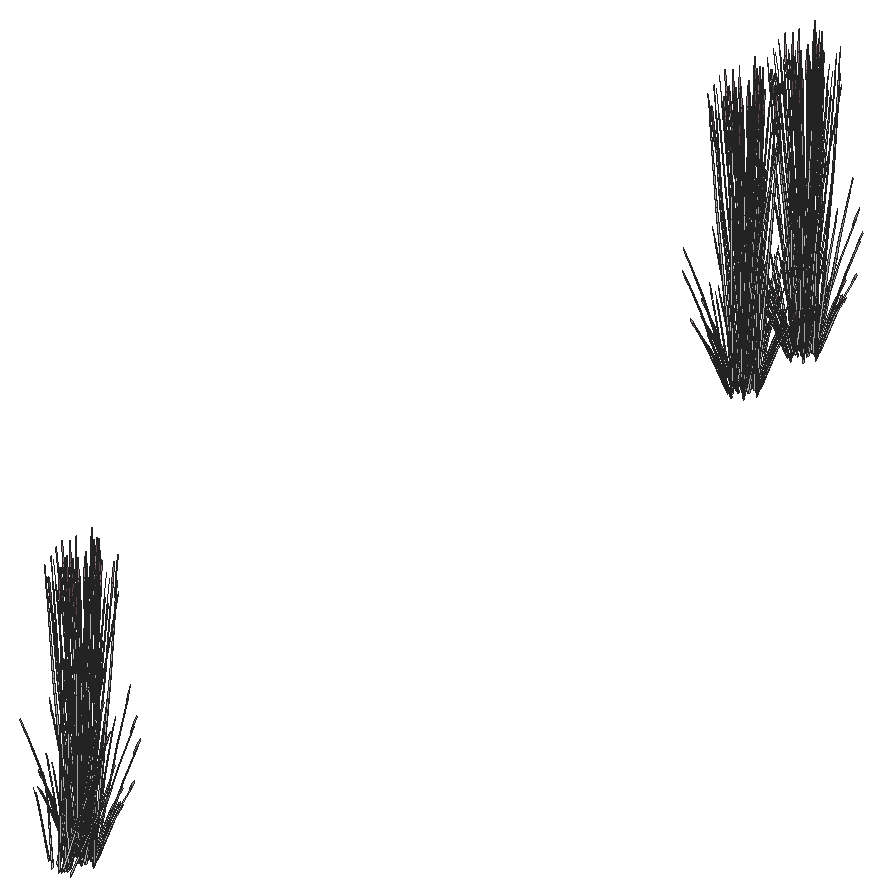
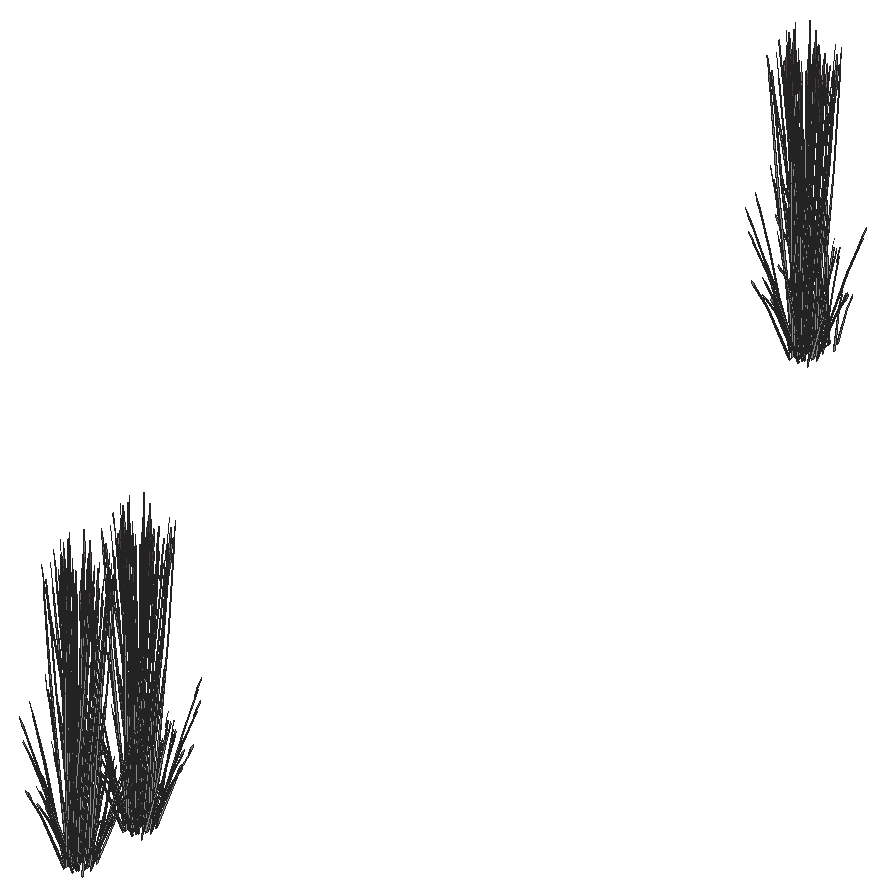
# SketchUp Ruby script. Lengths in inches.
U = 1.inch
M = Sketchup.active_model
def pt(a) = Geom::Point3d.new(a.map { |v| v * U })
def face(e, loops, mat)
  f = e.add_face(loops[0].map { |a| pt(a) })
  loops[1..].each { |l| e.add_face(l.map { |a| pt(a) }).erase! }
  f.material = f.back_material = mat if mat
  f
end
# faces: each face lists its corners as indices into pts; further lists are holes
def faces(e, pts, list, mat = nil) = list.each { |f| face(e, (f[0].is_a?(Array) ? f : [f]).map { |l| l.map { |i| pts[i] } }, mat) }
# xy, xz, yz: faces in a plane at the given z, y or x. An outline is a flat list of corners, or four numbers for a rectangle; further outlines are holes
def ring(l) = l.size == 4 ? [[l[0], l[1]], [l[2], l[1]], [l[2], l[3]], [l[0], l[3]]] : l.each_slice(2).to_a
def flat(e, list, mat, &to3) = list.each { |f| face(e, (f[0].is_a?(Array) ? f : [f]).map { |l| ring(l).map { |u, v| to3.(u, v) } }, mat) }
def xy(e, z, list, mat = nil) = flat(e, list, mat) { |x, y| [x, y, z] }
def xz(e, y, list, mat = nil) = flat(e, list, mat) { |x, z| [x, y, z] }
def yz(e, x, list, mat = nil) = flat(e, list, mat) { |y, z| [x, y, z] }
def lines(e, pts, list) = list.each { |a, b| e.add_line(pt(pts[a]), pt(pts[b])) }
# prism: a flat outline (further loops are holes) pulled along v
def prism(e, loops, v, mat = nil)
  f = face(e, loops, mat); d = Geom::Vector3d.new(v.map { |x| x * U })
  f.pushpull(f.normal.samedirection?(d) ? d.length : -d.length)
end
def box(e, o, s, mat = nil) = prism(e, [[o, [o[0] + s[0], o[1], o[2]], [o[0] + s[0], o[1] + s[1], o[2]], [o[0], o[1] + s[1], o[2]]]], [0, 0, s[2]], mat)
def at(x, y, z, deg = 0) = Geom::Transformation.translation(pt([x, y, z])) * Geom::Transformation.rotation(ORIGIN, Z_AXIS, deg.degrees)
def axes(o, x, y, z) = Geom::Transformation.new([*x, 0, *y, 0, *z, 0, *pt(o).to_a, 1])
def part(name) = M.definitions.add(name)
# library, detail: a bought-in or finely detailed component or shape, given as its bounding box
def library(name, o, s) = part(name).tap { |d| box(d.entities, o, s) }
def detail(e, o, s) = box(e.add_group.entities, o, s)
def put(e, d, t, mat = nil) = e.add_instance(d, t).tap { |i| i.material = mat if mat }
def group(e, t, mat = nil) = e.add_group.tap { |g| g.transformation = t; g.material = mat if mat }.entities
root = M.entities
M.materials.add("LightPink_Translucent").color = [144, 107, 117]
M.materials["LightPink_Translucent"].alpha = 0.75
c1 = part("blade")
p = [[2.15,0.21,22],[0,0.17,0],[0.09,0.45,0],[2.18,0.31,22],[2.29,0.31,22],[0.38,0.45,0],
  [2.48,0.24,33],[2.49,0.24,33],[2.48,0.22,33]]
faces(c1.entities,p,[[0,1,2,3],[4,5,2,3],[6,3,4,7],[8,0,3,6]])
c2 = part("seeds")
p = [[0.3,-0.1,1.38],[-0.01,-0.03,1.59],[-0.01,-0.03,0.03],[0.14,-0.07,-0.07],[0.29,-0.03,3],[0.15,0.01,3.11]]
faces(c2.entities,p,[[0,1,2,3],[1,0,4,5]],"LightPink_Translucent")
c3 = part("blade with seeds")
put(c3.entities,c1,at(0,0,0))
put(c3.entities,c2,axes([2.4,0.25,30.99],[1.5799,-0.05474,1.17369],[-0.12525,1.92788,0.29478],[-0.07173,-0.02425,1.56792]))
put(root,c3,axes([426.58,488.27,152.34],[0.17079,-0.21377,0.97034],[0.06739,0.33841,0.71294],[-0.12342,0.0606,0.21373]))
put(root,c3,axes([428.38,490.95,152],[-0.25622,-0.47263,0],[0.42866,-0.26357,-0.43598],[0.09763,-0.06003,1.38303]))
put(root,c3,axes([429.57,487.08,152.25],[0.04775,0.53819,-0.2458],[-0.49736,0.03254,-0.42242],[-0.08758,0.07169,1.34921]))
put(root,c3,axes([428.95,490.38,151.8],[-0.28319,0.27058,-0.03288],[-0.25948,-0.29635,-0.1491],[-0.01827,-0.08397,0.4918]))
put(root,c3,axes([429.76,488.09,151.97],[0.51304,0.1533,0.25983],[-0.12835,0.54797,-0.30828],[-0.08491,0.06858,1.39295]))
put(root,c3,axes([431.01,491.7,152.1875],[-0.1464,-0.01397,1.20808],[-0.14998,-0.37477,-0.25981],[0.17985,-0.10602,0.51652]))
put(root,c3,axes([431.18,491.01,152.34],[-0.1365,0.2401,0.97034],[-0.11733,-0.32258,0.71294],[0.11274,-0.08083,0.21373]))
put(root,c3,axes([430.42,488.04,152.34],[-0.23074,-0.13562,0.97034],[0.29794,-0.1378,0.71294],[0.08036,0.11673,0.21373]))
put(root,c3,axes([428.89,492.26,152.25],[-0.04775,-0.53819,-0.2458],[0.49736,-0.03254,-0.42242],[0.08758,-0.07169,1.34921]))
put(root,c3,axes([430.08,488.39,152],[0.25622,0.47263,0],[-0.42866,0.26357,-0.43598],[-0.09763,0.06003,1.38303]))
put(root,c3,axes([427.54,490.875,151.8],[-0.11822,0.38513,-0.03288],[-0.36385,-0.11847,-0.1491],[-0.05524,-0.06299,0.4918]))
put(root,c3,axes([430.48,488.55,151.26],[0.02986,-0.06809,1.48974],[0.37589,-0.20055,-0.22758],[0.11396,0.1038,0.25375]))
put(root,c3,axes([428.66,492.82,152.25],[-0.46151,-0.22505,-0.2458],[0.22222,-0.475,-0.42242],[-0.0145,-0.11662,1.34921]))
put(root,c3,axes([429.86,486.52,152.4],[-0.01119,-0.44408,1.19347],[0.50665,0.11511,0.50532],[-0.11983,0.243,1.12654]))
put(root,c3,axes([427.03,488.49,151.26],[0.05497,0.04712,1.48974],[0.09321,0.43661,-0.22758],[-0.12183,0.0931,0.25375]))
put(root,c3,axes([427.34,492.63,152],[-0.51243,0,0],[0,-0.52715,-0.43598],[0,-0.12006,1.38303]))
put(root,c3,axes([427.43,491.69,152.1875],[0.08001,0.13132,1.20808],[-0.18437,0.35694,-0.25981],[-0.18931,-0.08532,0.51652]))
put(root,c3,axes([430.46,488.66,152.25],[-0.26279,-0.01479,0.88755],[0.17355,-0.31417,0.49003],[0.10382,0.11162,0.6962]))
put(root,c3,axes([427.74,492.5,151.97],[-0.38118,0.39654,0.25983],[-0.38142,-0.39237,-0.30828],[-0.01331,-0.11261,1.39295]))
put(root,c3,axes([429.6,487.9,152.1875],[0.00723,-0.15635,1.20808],[0.34559,-0.17464,-0.25981],[0.10668,0.18713,0.51652]))
put(root,c3,axes([428.95,492.68,152.06],[0.46174,0.2286,0.2033],[-0.22222,0.475,0.42242],[0,-0.1095,1.35626]))
put(root,c3,axes([428.77,493.32,152.06],[0.10862,-0.55889,-0.19793],[0.515,0.09742,0.43313],[-0.08999,-0.07718,1.32161]))
put(root,c3,axes([428.03,489.2,152.34],[-0.01061,-0.28045,0.97034],[0.26501,0.20003,0.71294],[-0.05212,0.13367,0.21373]))
put(root,c3,axes([426.95,492.09,152.34],[0.26163,-0.03375,0.97034],[-0.16596,0.29737,0.71294],[-0.12929,-0.04461,0.21373]))
put(root,c3,axes([428.73,488.53,151.26],[0.06632,-0.02567,1.48974],[0.39894,0.14126,-0.22758],[0.01167,0.15921,0.25375]))
put(root,c3,axes([428.8,492.36,152.3],[-0.44501,0.02912,0.37796],[-0.04024,-0.48332,-0.1819],[0.07967,-0.04899,1.2135]))
put(root,c3,axes([427.65,492.71,152.09],[0,0.47166,0.41945],[-0.45849,0,0],[0,-0.10742,1.33059]))
put(root,c3,axes([430.27,491.07,152.01],[0.25622,-0.47263,0],[0.42866,0.26357,-0.43598],[0.09763,0.06003,1.38303]))
put(root,c3,axes([428.79,492.54,151.99],[0.17817,0.52741,0.38653],[-0.50909,0.1834,0.15168],[0.00622,-0.09691,1.34202]))
put(root,c3,axes([427.8125,488.6,152.38],[0.37228,-0.08352,0.05498],[0.08559,0.3365,-0.7291],[-0.0236,0.17034,0.65354]))
put(root,c3,axes([431.28,492.94,151.67],[-0.26394,0.0566,1.1961],[-0.04201,-0.45055,0.06846],[0.18486,-0.06819,0.68062]))
put(root,c3,axes([431.76,492.54,151.91],[-0.25407,-0.3016,-0.05481],[0.27826,-0.27635,-0.2485],[0.07884,-0.01946,0.81966]))
put(root,c3,axes([428.7,492.95,152.3],[-0.19883,0.425,0.37796],[-0.41314,-0.20454,-0.1819],[0,-0.09797,1.2135]))
put(root,c3,axes([429.43,492.58,151.86],[0,-0.54574,0],[0.51243,0,0],[0,0,1.51605]))
put(root,c3,axes([430.05,491.32,152.09],[-0.38354,-0.23583,0.41945],[0.22925,-0.42288,0],[0.08735,0.05371,1.33059]))
put(root,c3,axes([429.18,492.24,151.99],[-0.33979,0.42804,0.38653],[-0.40368,-0.37784,0.15168],[0.08192,-0.04272,1.34202]))
put(root,c3,axes([429.56,493,151.94],[-0.38118,-0.40596,-0.0518],[0.38142,-0.40621,0],[-0.01331,-0.01418,1.48322]))
put(root,c3,axes([428.59,491.53,152.09],[-0.11838,0.46875,0.14904],[-0.43321,-0.13265,0.29641],[0.07483,-0.00228,1.35512]))
put(root,c3,axes([428.42,491.91,151.35],[-0.40337,0.18883,1.08919],[-0.12839,-0.54182,0.42321],[0.24769,0.00901,1.23883]))
put(root,c3,axes([429.5,492.05,152.21],[0.07906,-0.42093,0.12232],[0.38625,0.07307,-0.3493],[0.07029,0.04322,1.07074]))
put(root,c3,axes([428.83,493.05,151.99],[0.51796,0.09937,0.38653],[-0.10541,0.56124,0.15168],[-0.07569,-0.05419,1.34202]))
put(root,c3,axes([431.57,492.65,151.26],[-0.02142,-0.07161,1.48974],[0.14855,-0.41887,-0.22758],[0.14984,-0.00603,0.25375]))
put(root,c3,axes([427.14,492.57,151.26],[0.01039,0.07433,1.48974],[-0.20952,0.38819,-0.22758],[-0.14882,-0.01957,0.25375]))
put(root,c3,axes([427.72,488.95,152.1875],[0.12932,-0.07441,1.20808],[0.31929,0.22435,-0.25981],[-0.09503,0.19413,0.51652]))
put(root,c3,axes([429.33,492.16,152.3],[-0.24618,-0.39589,0.37796],[0.37289,-0.27878,-0.1819],[0.07967,0.04899,1.2135]))
put(root,c3,axes([428.55,493.95,152.09],[0.44036,-0.12519,0.14904],[0.10874,0.46588,0.29641],[-0.03927,-0.06788,1.35512]))
put(root,c3,axes([429.46,492.19,152.25],[0.41376,-0.31314,-0.2458],[0.27514,0.44246,-0.42242],[0.10209,0.04493,1.34921]))
put(root,c3,axes([429.78,492.7,151.86],[0.45849,0,0],[0,0.4883,0],[0,0,1.50718]))
put(root,c3,axes([429,493.32,152.25],[-0.41376,0.31314,-0.2458],[-0.27514,-0.44246,-0.42242],[-0.10209,-0.04493,1.34921]))
put(root,c3,axes([429.91,491.56,152.09],[-0.44036,0.12519,0.14904],[-0.10874,-0.46588,0.29641],[0.03927,0.06788,1.35512]))
put(root,c3,axes([429.63,492.45,152.01],[-0.51796,-0.09937,0.41563],[0.10541,-0.56124,0.1631],[0.07569,0.05419,1.44303]))
put(root,c3,axes([429.21,493.84,151.86],[-0.13371,-0.40664,0],[0.38182,-0.1424,0],[0,0,1.30413]))
put(root,c3,axes([428.96,493.45,152.21],[-0.07906,0.42093,0.12232],[-0.38625,-0.07307,-0.3493],[-0.07029,-0.04322,1.07074]))
put(root,c3,axes([429.71,493.78,151.85],[0.43024,-0.16003,-0.16218],[0.15118,0.46099,0.00007],[0.04749,-0.01769,1.46908]))
put(root,c3,axes([429.86,493.98,152.09],[0.11838,-0.46875,0.14904],[0.43321,0.13265,0.29641],[-0.07483,0.00228,1.35512]))
put(root,c3,axes([429.77,492.91,151.87],[0.28606,0.30466,0],[-0.28606,0.30466,0],[0,0,1.42996]))
put(root,c3,axes([430.54,492.78,152.09],[-0.32198,-0.34356,0.14904],[0.32447,-0.33323,0.29641],[-0.03556,0.07016,1.35512]))
put(root,c3,axes([431.83,493.09,152.34],[-0.2532,0.07787,0.97034],[0.11918,-0.32181,0.71294],[0.13432,0.02202,0.21373]))
put(root,c3,axes([429.12,494.02,151.86],[-0.41314,-0.21175,0],[0.19883,-0.43999,0],[0,0,1.37455]))
put(root,c3,axes([429.46,493.46,152.08],[-0.40016,-0.37963,-0.21282],[0.33672,-0.42629,0.46574],[-0.10776,0.04441,1.42109]))
put(root,c3,axes([428.41,494.1875,152.09],[0.38354,0.23583,0.41945],[-0.22925,0.42288,0],[-0.08735,-0.05371,1.33059]))
put(root,c3,axes([429.76,492.56,152.3],[0.19883,-0.425,0.37796],[0.41314,0.20454,-0.1819],[0,0.09797,1.2135]))
put(root,c3,axes([429.68,492.8,151.9375],[0,0.54548,-0.04762],[-0.51243,0,0],[0,0.01714,1.5153]))
put(root,c3,axes([428.1875,494.43,152],[-0.25622,0.47263,0],[-0.42866,-0.26357,-0.43598],[-0.09763,-0.06003,1.38303]))
put(root,c3,axes([430.8,492.79,152.09],[0,-0.47166,0.41945],[0.45849,0,0],[0,0.10742,1.33059]))
put(root,c3,axes([429.66,493.15,152.3],[0.44501,-0.02912,0.37796],[0.04024,0.48332,-0.1819],[-0.07967,0.04899,1.2135]))
put(root,c3,axes([429.93,492.65,152.21],[0.38182,-0.13755,0.12232],[0.13371,0.39278,-0.3493],[0,0.08644,1.07074]))
put(root,c3,axes([431.35,493.61,152.1875],[-0.0987,-0.116,1.20808],[0.12841,-0.38374,-0.25981],[0.19968,0.05198,0.51652]))
put(root,c3,axes([429.59,494.03,151.86],[0.41314,0.21175,0],[-0.19883,0.43999,0],[0,0,1.47801]))
put(root,c3,axes([429.75,494.5,151.85],[-0.25302,-0.47428,-0.04344],[0.42866,-0.26357,0.43598],[-0.10563,0.04516,1.38235]))
put(root,c3,axes([429.66,493.35,152.21],[0.30276,0.28338,0.12232],[-0.25254,0.31972,-0.3493],[-0.07029,0.04322,1.07074]))
put(root,c3,axes([429.99,494.23,152.09],[0.38354,-0.23583,0.41945],[0.22925,0.42288,0],[-0.08735,0.05371,1.33059]))
put(root,c3,axes([429.44,493.85,151.9375],[0.17817,0.54185,-0.05079],[-0.50909,0.18987,0],[0.00622,0.01892,1.45452]))
put(root,c3,axes([426.88,493.61,152.1875],[0.14242,0.03872,1.20808],[0.09179,0.39548,-0.25981],[-0.19345,0.07403,0.51652]))
put(root,c3,axes([431.12,492.87,152.01],[0.51243,0,0],[0,0.52715,-0.43598],[0,0.12006,1.38303]))
put(root,c3,axes([430.91,493.14,151.86],[-0.51218,-0.00377,-0.04204],[0,-0.52715,0.42192],[-0.0161,0.12,1.33776]))
put(root,c3,axes([429.8,492.68,152.25],[0.46151,0.22505,-0.2458],[-0.22222,0.475,-0.42242],[0.0145,0.11662,1.34921]))
put(root,c3,axes([426.58,494.44,152.34],[0.17079,-0.21377,0.97034],[0.06739,0.33841,0.71294],[-0.12342,0.0606,0.21373]))
put(root,c3,axes([429.57,493.25,152.25],[0.04775,0.53819,-0.2458],[-0.49736,0.03254,-0.42242],[-0.08758,0.07169,1.34921]))
put(root,c3,axes([429.76,494.26,151.97],[0.51304,0.1533,0.25983],[-0.12835,0.54797,-0.30828],[-0.08491,0.06858,1.39295]))
put(root,c3,axes([430.42,494.21,152.34],[-0.23074,-0.13562,0.97034],[0.29794,-0.1378,0.71294],[0.08036,0.11673,0.21373]))
put(root,c3,axes([430.08,494.55,152],[0.25622,0.47263,0],[-0.42866,0.26357,-0.43598],[-0.09763,0.06003,1.38303]))
put(root,c3,axes([430.48,494.71,151.26],[0.02986,-0.06809,1.48974],[0.37589,-0.20055,-0.22758],[0.11396,0.1038,0.25375]))
put(root,c3,axes([429.86,492.68,152.4],[-0.01119,-0.44408,1.19347],[0.50665,0.11511,0.50532],[-0.11983,0.243,1.12654]))
put(root,c3,axes([427.03,494.65,151.26],[0.05497,0.04712,1.48974],[0.09321,0.43661,-0.22758],[-0.12183,0.0931,0.25375]))
put(root,c3,axes([430.46,494.83,152.25],[-0.26279,-0.01479,0.88755],[0.17355,-0.31417,0.49003],[0.10382,0.11162,0.6962]))
put(root,c3,axes([429.6,494.0625,152.1875],[0.00723,-0.15635,1.20808],[0.34559,-0.17464,-0.25981],[0.10668,0.18713,0.51652]))
put(root,c3,axes([428.03,495.37,152.34],[-0.01061,-0.28045,0.97034],[0.26501,0.20003,0.71294],[-0.05212,0.13367,0.21373]))
put(root,c3,axes([428.73,494.7,151.26],[0.06632,-0.02567,1.48974],[0.39894,0.14126,-0.22758],[0.01167,0.15921,0.25375]))
put(root,c3,axes([427.8125,494.76,152.38],[0.37228,-0.08352,0.05498],[0.08559,0.3365,-0.7291],[-0.0236,0.17034,0.65354]))
put(root,c3,axes([427.72,495.12,152.1875],[0.12932,-0.07441,1.20808],[0.31929,0.22435,-0.25981],[-0.09503,0.19413,0.51652]))
put(root,c3,axes([417.88,660.26,152.1875],[-0.11649,0.09547,1.20808],[-0.34886,-0.1671,-0.25981],[0.06467,-0.20781,0.51652]))
put(root,c3,axes([416.08,660.08,152.1875],[-0.02482,0.15429,1.20808],[-0.36278,0.12916,-0.25981],[-0.0848,-0.19943,0.51652]))
put(root,c3,axes([417.02,659.74,151.26],[-0.06874,0.01699,1.48974],[-0.38012,-0.19128,-0.22758],[0.00638,-0.15955,0.25375]))
put(root,c3,axes([417.46,659.5,152.34],[0.05257,0.27504,0.97034],[-0.29163,-0.15233,0.71294],[0.03138,-0.14083,0.21373]))
put(root,c3,axes([415.96,659.83,152.34],[0.21377,0.16416,0.97034],[-0.31132,0.09868,0.71294],[-0.06661,-0.12616,0.21373]))
put(root,c3,axes([415.79,660.32,151.26],[-0.0397,0.06213,1.48974],[-0.40116,0.13396,-0.22758],[-0.09691,-0.12186,0.25375]))
put(root,c3,axes([418.7,660.55,151.26],[-0.06134,-0.03716,1.48974],[-0.15755,-0.41512,-0.22758],[0.10629,-0.11265,0.25375]))
put(root,c3,axes([416.38,660.64,152],[-0.25622,-0.47263,0],[0.42866,-0.26357,-0.43598],[0.09763,-0.06003,1.38303]))
put(root,c3,axes([416.95,660.07,151.8],[-0.28319,0.27058,-0.03288],[-0.25948,-0.29635,-0.1491],[-0.01827,-0.08397,0.4918]))
put(root,c3,axes([419.01,661.38,152.1875],[-0.1464,-0.01397,1.20808],[-0.14998,-0.37477,-0.25981],[0.17985,-0.10602,0.51652]))
put(root,c3,axes([419.18,660.69,152.34],[-0.1365,0.2401,0.97034],[-0.11733,-0.32258,0.71294],[0.11274,-0.08083,0.21373]))
put(root,c3,axes([416.89,661.94,152.25],[-0.04775,-0.53819,-0.2458],[0.49736,-0.03254,-0.42242],[0.08758,-0.07169,1.34921]))
put(root,c3,axes([415.54,660.5625,151.8],[-0.11822,0.38513,-0.03288],[-0.36385,-0.11847,-0.1491],[-0.05524,-0.06299,0.4918]))
put(root,c3,axes([416.66,662.51,152.25],[-0.46151,-0.22505,-0.2458],[0.22222,-0.475,-0.42242],[-0.0145,-0.11662,1.34921]))
put(root,c3,axes([415.34,662.32,152],[-0.51243,0,0],[0,-0.52715,-0.43598],[0,-0.12006,1.38303]))
put(root,c3,axes([415.43,661.38,152.1875],[0.08001,0.13132,1.20808],[-0.18437,0.35694,-0.25981],[-0.18931,-0.08532,0.51652]))
put(root,c3,axes([415.74,662.18,151.97],[-0.38118,0.39654,0.25983],[-0.38142,-0.39237,-0.30828],[-0.01331,-0.11261,1.39295]))
put(root,c3,axes([416.95,662.37,152.06],[0.46174,0.2286,0.2033],[-0.22222,0.475,0.42242],[0,-0.1095,1.35626]))
put(root,c3,axes([416.77,663.01,152.06],[0.10862,-0.55889,-0.19793],[0.515,0.09742,0.43313],[-0.08999,-0.07718,1.32161]))
put(root,c3,axes([414.95,661.77,152.34],[0.26163,-0.03375,0.97034],[-0.16596,0.29737,0.71294],[-0.12929,-0.04461,0.21373]))
put(root,c3,axes([416.8,662.05,152.3],[-0.44501,0.02912,0.37796],[-0.04024,-0.48332,-0.1819],[0.07967,-0.04899,1.2135]))
put(root,c3,axes([415.65,662.4,152.09],[0,0.47166,0.41945],[-0.45849,0,0],[0,-0.10742,1.33059]))
put(root,c3,axes([418.27,660.76,152.01],[0.25622,-0.47263,0],[0.42866,0.26357,-0.43598],[0.09763,0.06003,1.38303]))
put(root,c3,axes([416.79,662.22,151.99],[0.17817,0.52741,0.38653],[-0.50909,0.1834,0.15168],[0.00622,-0.09691,1.34202]))
put(root,c3,axes([419.28,662.625,151.67],[-0.26394,0.0566,1.1961],[-0.04201,-0.45055,0.06846],[0.18486,-0.06819,0.68062]))
put(root,c3,axes([419.76,662.23,151.91],[-0.25407,-0.3016,-0.05481],[0.27826,-0.27635,-0.2485],[0.07884,-0.01946,0.81966]))
put(root,c3,axes([416.7,662.64,152.3],[-0.19883,0.425,0.37796],[-0.41314,-0.20454,-0.1819],[0,-0.09797,1.2135]))
put(root,c3,axes([417.43,662.27,151.86],[0,-0.54574,0],[0.51243,0,0],[0,0,1.51605]))
put(root,c3,axes([418.05,661,152.09],[-0.38354,-0.23583,0.41945],[0.22925,-0.42288,0],[0.08735,0.05371,1.33059]))
put(root,c3,axes([417.18,661.92,151.99],[-0.33979,0.42804,0.38653],[-0.40368,-0.37784,0.15168],[0.08192,-0.04272,1.34202]))
put(root,c3,axes([417.56,662.6875,151.94],[-0.38118,-0.40596,-0.0518],[0.38142,-0.40621,0],[-0.01331,-0.01418,1.48322]))
put(root,c3,axes([416.59,661.22,152.09],[-0.11838,0.46875,0.14904],[-0.43321,-0.13265,0.29641],[0.07483,-0.00228,1.35512]))
put(root,c3,axes([416.42,661.6,151.35],[-0.40337,0.18883,1.08919],[-0.12839,-0.54182,0.42321],[0.24769,0.00901,1.23883]))
put(root,c3,axes([417.5,661.74,152.21],[0.07906,-0.42093,0.12232],[0.38625,0.07307,-0.3493],[0.07029,0.04322,1.07074]))
put(root,c3,axes([416.83,662.74,151.99],[0.51796,0.09937,0.38653],[-0.10541,0.56124,0.15168],[-0.07569,-0.05419,1.34202]))
put(root,c3,axes([419.57,662.33,151.26],[-0.02142,-0.07161,1.48974],[0.14855,-0.41887,-0.22758],[0.14984,-0.00603,0.25375]))
put(root,c3,axes([415.14,662.26,151.26],[0.01039,0.07433,1.48974],[-0.20952,0.38819,-0.22758],[-0.14882,-0.01957,0.25375]))
put(root,c3,axes([417.33,661.85,152.3],[-0.24618,-0.39589,0.37796],[0.37289,-0.27878,-0.1819],[0.07967,0.04899,1.2135]))
put(root,c3,axes([416.55,663.63,152.09],[0.44036,-0.12519,0.14904],[0.10874,0.46588,0.29641],[-0.03927,-0.06788,1.35512]))
put(root,c3,axes([417.46,661.875,152.25],[0.41376,-0.31314,-0.2458],[0.27514,0.44246,-0.42242],[0.10209,0.04493,1.34921]))
put(root,c3,axes([417.78,662.39,151.86],[0.45849,0,0],[0,0.4883,0],[0,0,1.50718]))
put(root,c3,axes([417,663,152.25],[-0.41376,0.31314,-0.2458],[-0.27514,-0.44246,-0.42242],[-0.10209,-0.04493,1.34921]))
put(root,c3,axes([417.91,661.24,152.09],[-0.44036,0.12519,0.14904],[-0.10874,-0.46588,0.29641],[0.03927,0.06788,1.35512]))
put(root,c3,axes([417.63,662.14,152.01],[-0.51796,-0.09937,0.41563],[0.10541,-0.56124,0.1631],[0.07569,0.05419,1.44303]))
put(root,c3,axes([417.21,663.52,151.86],[-0.13371,-0.40664,0],[0.38182,-0.1424,0],[0,0,1.30413]))
put(root,c3,axes([416.96,663.14,152.21],[-0.07906,0.42093,0.12232],[-0.38625,-0.07307,-0.3493],[-0.07029,-0.04322,1.07074]))
put(root,c3,axes([417.71,663.47,151.85],[0.43024,-0.16003,-0.16218],[0.15118,0.46099,0.00007],[0.04749,-0.01769,1.46908]))
put(root,c3,axes([417.86,663.66,152.09],[0.11838,-0.46875,0.14904],[0.43321,0.13265,0.29641],[-0.07483,0.00228,1.35512]))
put(root,c3,axes([417.77,662.6,151.87],[0.28606,0.30466,0],[-0.28606,0.30466,0],[0,0,1.42996]))
put(root,c3,axes([418.54,662.46,152.09],[-0.32198,-0.34356,0.14904],[0.32447,-0.33323,0.29641],[-0.03556,0.07016,1.35512]))
put(root,c3,axes([419.83,662.78,152.34],[-0.2532,0.07787,0.97034],[0.11918,-0.32181,0.71294],[0.13432,0.02202,0.21373]))
put(root,c3,axes([417.12,663.71,151.86],[-0.41314,-0.21175,0],[0.19883,-0.43999,0],[0,0,1.37455]))
put(root,c3,axes([417.46,663.14,152.08],[-0.40016,-0.37963,-0.21282],[0.33672,-0.42629,0.46574],[-0.10776,0.04441,1.42109]))
put(root,c3,axes([416.41,663.87,152.09],[0.38354,0.23583,0.41945],[-0.22925,0.42288,0],[-0.08735,-0.05371,1.33059]))
put(root,c3,axes([417.76,662.24,152.3],[0.19883,-0.425,0.37796],[0.41314,0.20454,-0.1819],[0,0.09797,1.2135]))
put(root,c3,axes([417.68,662.48,151.9375],[0,0.54548,-0.04762],[-0.51243,0,0],[0,0.01714,1.5153]))
put(root,c3,axes([416.1875,664.12,152],[-0.25622,0.47263,0],[-0.42866,-0.26357,-0.43598],[-0.09763,-0.06003,1.38303]))
put(root,c3,axes([418.8,662.48,152.09],[0,-0.47166,0.41945],[0.45849,0,0],[0,0.10742,1.33059]))
put(root,c3,axes([417.66,662.83,152.3],[0.44501,-0.02912,0.37796],[0.04024,0.48332,-0.1819],[-0.07967,0.04899,1.2135]))
put(root,c3,axes([417.93,662.34,152.21],[0.38182,-0.13755,0.12232],[0.13371,0.39278,-0.3493],[0,0.08644,1.07074]))
put(root,c3,axes([419.35,663.29,152.1875],[-0.0987,-0.116,1.20808],[0.12841,-0.38374,-0.25981],[0.19968,0.05198,0.51652]))
put(root,c3,axes([417.59,663.72,151.86],[0.41314,0.21175,0],[-0.19883,0.43999,0],[0,0,1.47801]))
put(root,c3,axes([417.75,664.19,151.85],[-0.25302,-0.47428,-0.04344],[0.42866,-0.26357,0.43598],[-0.10563,0.04516,1.38235]))
put(root,c3,axes([417.66,663.04,152.21],[0.30276,0.28338,0.12232],[-0.25254,0.31972,-0.3493],[-0.07029,0.04322,1.07074]))
put(root,c3,axes([417.99,663.91,152.09],[0.38354,-0.23583,0.41945],[0.22925,0.42288,0],[-0.08735,0.05371,1.33059]))
put(root,c3,axes([417.44,663.54,151.9375],[0.17817,0.54185,-0.05079],[-0.50909,0.18987,0],[0.00622,0.01892,1.45452]))
put(root,c3,axes([414.88,663.29,152.1875],[0.14242,0.03872,1.20808],[0.09179,0.39548,-0.25981],[-0.19345,0.07403,0.51652]))
put(root,c3,axes([419.12,662.56,152.01],[0.51243,0,0],[0,0.52715,-0.43598],[0,0.12006,1.38303]))
put(root,c3,axes([418.91,662.83,151.86],[-0.51218,-0.00377,-0.04204],[0,-0.52715,0.42192],[-0.0161,0.12,1.33776]))
put(root,c3,axes([417.8,662.37,152.25],[0.46151,0.22505,-0.2458],[-0.22222,0.475,-0.42242],[0.0145,0.11662,1.34921]))
put(root,c3,axes([414.58,664.12,152.34],[0.17079,-0.21377,0.97034],[0.06739,0.33841,0.71294],[-0.12342,0.0606,0.21373]))
put(root,c3,axes([417.57,662.93,152.25],[0.04775,0.53819,-0.2458],[-0.49736,0.03254,-0.42242],[-0.08758,0.07169,1.34921]))
put(root,c3,axes([417.76,663.94,151.97],[0.51304,0.1533,0.25983],[-0.12835,0.54797,-0.30828],[-0.08491,0.06858,1.39295]))
put(root,c3,axes([418.42,663.89,152.34],[-0.23074,-0.13562,0.97034],[0.29794,-0.1378,0.71294],[0.08036,0.11673,0.21373]))
put(root,c3,axes([418.08,664.24,152],[0.25622,0.47263,0],[-0.42866,0.26357,-0.43598],[-0.09763,0.06003,1.38303]))
put(root,c3,axes([418.48,664.4,151.26],[0.02986,-0.06809,1.48974],[0.37589,-0.20055,-0.22758],[0.11396,0.1038,0.25375]))
put(root,c3,axes([417.86,662.37,152.4],[-0.01119,-0.44408,1.19347],[0.50665,0.11511,0.50532],[-0.11983,0.243,1.12654]))
put(root,c3,axes([415.03,664.34,151.26],[0.05497,0.04712,1.48974],[0.09321,0.43661,-0.22758],[-0.12183,0.0931,0.25375]))
put(root,c3,axes([418.46,664.51,152.25],[-0.26279,-0.01479,0.88755],[0.17355,-0.31417,0.49003],[0.10382,0.11162,0.6962]))
put(root,c3,axes([417.6,663.75,152.1875],[0.00723,-0.15635,1.20808],[0.34559,-0.17464,-0.25981],[0.10668,0.18713,0.51652]))
put(root,c3,axes([416.03,665.05,152.34],[-0.01061,-0.28045,0.97034],[0.26501,0.20003,0.71294],[-0.05212,0.13367,0.21373]))
put(root,c3,axes([416.73,664.38,151.26],[0.06632,-0.02567,1.48974],[0.39894,0.14126,-0.22758],[0.01167,0.15921,0.25375]))
put(root,c3,axes([415.8125,664.45,152.38],[0.37228,-0.08352,0.05498],[0.08559,0.3365,-0.7291],[-0.0236,0.17034,0.65354]))
put(root,c3,axes([415.72,664.8,152.1875],[0.12932,-0.07441,1.20808],[0.31929,0.22435,-0.25981],[-0.09503,0.19413,0.51652]))
put(root,c3,axes([417.88,674.13,152.1875],[-0.11649,0.09547,1.20808],[-0.34886,-0.1671,-0.25981],[0.06467,-0.20781,0.51652]))
put(root,c3,axes([416.08,673.95,152.1875],[-0.02482,0.15429,1.20808],[-0.36278,0.12916,-0.25981],[-0.0848,-0.19943,0.51652]))
put(root,c3,axes([417.02,673.61,151.26],[-0.06874,0.01699,1.48974],[-0.38012,-0.19128,-0.22758],[0.00638,-0.15955,0.25375]))
put(root,c3,axes([417.46,673.375,152.34],[0.05257,0.27504,0.97034],[-0.29163,-0.15233,0.71294],[0.03138,-0.14083,0.21373]))
put(root,c3,axes([415.96,673.7,152.34],[0.21377,0.16416,0.97034],[-0.31132,0.09868,0.71294],[-0.06661,-0.12616,0.21373]))
put(root,c3,axes([415.79,674.2,151.26],[-0.0397,0.06213,1.48974],[-0.40116,0.13396,-0.22758],[-0.09691,-0.12186,0.25375]))
put(root,c3,axes([418.7,674.43,151.26],[-0.06134,-0.03716,1.48974],[-0.15755,-0.41512,-0.22758],[0.10629,-0.11265,0.25375]))
put(root,c3,axes([416.38,674.52,152],[-0.25622,-0.47263,0],[0.42866,-0.26357,-0.43598],[0.09763,-0.06003,1.38303]))
put(root,c3,axes([416.95,673.95,151.8],[-0.28319,0.27058,-0.03288],[-0.25948,-0.29635,-0.1491],[-0.01827,-0.08397,0.4918]))
put(root,c3,axes([419.01,675.26,152.1875],[-0.1464,-0.01397,1.20808],[-0.14998,-0.37477,-0.25981],[0.17985,-0.10602,0.51652]))
put(root,c3,axes([419.18,674.57,152.34],[-0.1365,0.2401,0.97034],[-0.11733,-0.32258,0.71294],[0.11274,-0.08083,0.21373]))
put(root,c3,axes([416.89,675.82,152.25],[-0.04775,-0.53819,-0.2458],[0.49736,-0.03254,-0.42242],[0.08758,-0.07169,1.34921]))
put(root,c3,axes([415.54,674.4375,151.8],[-0.11822,0.38513,-0.03288],[-0.36385,-0.11847,-0.1491],[-0.05524,-0.06299,0.4918]))
put(root,c3,axes([416.66,676.38,152.25],[-0.46151,-0.22505,-0.2458],[0.22222,-0.475,-0.42242],[-0.0145,-0.11662,1.34921]))
put(root,c3,axes([415.34,676.2,152],[-0.51243,0,0],[0,-0.52715,-0.43598],[0,-0.12006,1.38303]))
put(root,c3,axes([415.43,675.25,152.1875],[0.08001,0.13132,1.20808],[-0.18437,0.35694,-0.25981],[-0.18931,-0.08532,0.51652]))
put(root,c3,axes([415.74,676.06,151.97],[-0.38118,0.39654,0.25983],[-0.38142,-0.39237,-0.30828],[-0.01331,-0.11261,1.39295]))
put(root,c3,axes([416.95,676.24,152.06],[0.46174,0.2286,0.2033],[-0.22222,0.475,0.42242],[0,-0.1095,1.35626]))
put(root,c3,axes([416.77,676.88,152.06],[0.10862,-0.55889,-0.19793],[0.515,0.09742,0.43313],[-0.08999,-0.07718,1.32161]))
put(root,c3,axes([414.95,675.65,152.34],[0.26163,-0.03375,0.97034],[-0.16596,0.29737,0.71294],[-0.12929,-0.04461,0.21373]))
put(root,c3,axes([416.8,675.92,152.3],[-0.44501,0.02912,0.37796],[-0.04024,-0.48332,-0.1819],[0.07967,-0.04899,1.2135]))
put(root,c3,axes([415.65,676.28,152.09],[0,0.47166,0.41945],[-0.45849,0,0],[0,-0.10742,1.33059]))
put(root,c3,axes([418.27,674.63,152.01],[0.25622,-0.47263,0],[0.42866,0.26357,-0.43598],[0.09763,0.06003,1.38303]))
put(root,c3,axes([416.79,676.1,151.99],[0.17817,0.52741,0.38653],[-0.50909,0.1834,0.15168],[0.00622,-0.09691,1.34202]))
put(root,c3,axes([419.28,676.5,151.67],[-0.26394,0.0566,1.1961],[-0.04201,-0.45055,0.06846],[0.18486,-0.06819,0.68062]))
put(root,c3,axes([419.76,676.1,151.91],[-0.25407,-0.3016,-0.05481],[0.27826,-0.27635,-0.2485],[0.07884,-0.01946,0.81966]))
put(root,c3,axes([416.7,676.51,152.3],[-0.19883,0.425,0.37796],[-0.41314,-0.20454,-0.1819],[0,-0.09797,1.2135]))
put(root,c3,axes([417.43,676.14,151.86],[0,-0.54574,0],[0.51243,0,0],[0,0,1.51605]))
put(root,c3,axes([418.05,674.88,152.09],[-0.38354,-0.23583,0.41945],[0.22925,-0.42288,0],[0.08735,0.05371,1.33059]))
put(root,c3,axes([417.18,675.8,151.99],[-0.33979,0.42804,0.38653],[-0.40368,-0.37784,0.15168],[0.08192,-0.04272,1.34202]))
put(root,c3,axes([417.56,676.57,151.94],[-0.38118,-0.40596,-0.0518],[0.38142,-0.40621,0],[-0.01331,-0.01418,1.48322]))
put(root,c3,axes([416.59,675.09,152.09],[-0.11838,0.46875,0.14904],[-0.43321,-0.13265,0.29641],[0.07483,-0.00228,1.35512]))
put(root,c3,axes([416.42,675.47,151.35],[-0.40337,0.18883,1.08919],[-0.12839,-0.54182,0.42321],[0.24769,0.00901,1.23883]))
put(root,c3,axes([417.5,675.61,152.21],[0.07906,-0.42093,0.12232],[0.38625,0.07307,-0.3493],[0.07029,0.04322,1.07074]))
put(root,c3,axes([416.83,676.61,151.99],[0.51796,0.09937,0.38653],[-0.10541,0.56124,0.15168],[-0.07569,-0.05419,1.34202]))
put(root,c3,axes([419.57,676.21,151.26],[-0.02142,-0.07161,1.48974],[0.14855,-0.41887,-0.22758],[0.14984,-0.00603,0.25375]))
put(root,c3,axes([415.14,676.13,151.26],[0.01039,0.07433,1.48974],[-0.20952,0.38819,-0.22758],[-0.14882,-0.01957,0.25375]))
put(root,c3,axes([417.33,675.73,152.3],[-0.24618,-0.39589,0.37796],[0.37289,-0.27878,-0.1819],[0.07967,0.04899,1.2135]))
put(root,c3,axes([416.55,677.51,152.09],[0.44036,-0.12519,0.14904],[0.10874,0.46588,0.29641],[-0.03927,-0.06788,1.35512]))
put(root,c3,axes([417.46,675.75,152.25],[0.41376,-0.31314,-0.2458],[0.27514,0.44246,-0.42242],[0.10209,0.04493,1.34921]))
put(root,c3,axes([417.78,676.26,151.86],[0.45849,0,0],[0,0.4883,0],[0,0,1.50718]))
put(root,c3,axes([417,676.88,152.25],[-0.41376,0.31314,-0.2458],[-0.27514,-0.44246,-0.42242],[-0.10209,-0.04493,1.34921]))
put(root,c3,axes([417.91,675.12,152.09],[-0.44036,0.12519,0.14904],[-0.10874,-0.46588,0.29641],[0.03927,0.06788,1.35512]))
put(root,c3,axes([417.63,676.02,152.01],[-0.51796,-0.09937,0.41563],[0.10541,-0.56124,0.1631],[0.07569,0.05419,1.44303]))
put(root,c3,axes([417.21,677.4,151.86],[-0.13371,-0.40664,0],[0.38182,-0.1424,0],[0,0,1.30413]))
put(root,c3,axes([416.96,677.02,152.21],[-0.07906,0.42093,0.12232],[-0.38625,-0.07307,-0.3493],[-0.07029,-0.04322,1.07074]))
put(root,c3,axes([417.71,677.34,151.85],[0.43024,-0.16003,-0.16218],[0.15118,0.46099,0.00007],[0.04749,-0.01769,1.46908]))
put(root,c3,axes([417.86,677.54,152.09],[0.11838,-0.46875,0.14904],[0.43321,0.13265,0.29641],[-0.07483,0.00228,1.35512]))
put(root,c3,axes([417.77,676.47,151.87],[0.28606,0.30466,0],[-0.28606,0.30466,0],[0,0,1.42996]))
put(root,c3,axes([418.54,676.34,152.09],[-0.32198,-0.34356,0.14904],[0.32447,-0.33323,0.29641],[-0.03556,0.07016,1.35512]))
put(root,c3,axes([419.83,676.66,152.34],[-0.2532,0.07787,0.97034],[0.11918,-0.32181,0.71294],[0.13432,0.02202,0.21373]))
put(root,c3,axes([417.12,677.59,151.86],[-0.41314,-0.21175,0],[0.19883,-0.43999,0],[0,0,1.37455]))
put(root,c3,axes([417.46,677.02,152.08],[-0.40016,-0.37963,-0.21282],[0.33672,-0.42629,0.46574],[-0.10776,0.04441,1.42109]))
put(root,c3,axes([416.41,677.75,152.09],[0.38354,0.23583,0.41945],[-0.22925,0.42288,0],[-0.08735,-0.05371,1.33059]))
put(root,c3,axes([417.76,676.12,152.3],[0.19883,-0.425,0.37796],[0.41314,0.20454,-0.1819],[0,0.09797,1.2135]))
put(root,c3,axes([417.68,676.36,151.9375],[0,0.54548,-0.04762],[-0.51243,0,0],[0,0.01714,1.5153]))
put(root,c3,axes([416.1875,678,152],[-0.25622,0.47263,0],[-0.42866,-0.26357,-0.43598],[-0.09763,-0.06003,1.38303]))
put(root,c3,axes([418.8,676.35,152.09],[0,-0.47166,0.41945],[0.45849,0,0],[0,0.10742,1.33059]))
put(root,c3,axes([417.66,676.71,152.3],[0.44501,-0.02912,0.37796],[0.04024,0.48332,-0.1819],[-0.07967,0.04899,1.2135]))
put(root,c3,axes([417.93,676.21,152.21],[0.38182,-0.13755,0.12232],[0.13371,0.39278,-0.3493],[0,0.08644,1.07074]))
put(root,c3,axes([419.35,677.17,152.1875],[-0.0987,-0.116,1.20808],[0.12841,-0.38374,-0.25981],[0.19968,0.05198,0.51652]))
put(root,c3,axes([417.59,677.59,151.86],[0.41314,0.21175,0],[-0.19883,0.43999,0],[0,0,1.47801]))
put(root,c3,axes([417.75,678.0625,151.85],[-0.25302,-0.47428,-0.04344],[0.42866,-0.26357,0.43598],[-0.10563,0.04516,1.38235]))
put(root,c3,axes([417.66,676.91,152.21],[0.30276,0.28338,0.12232],[-0.25254,0.31972,-0.3493],[-0.07029,0.04322,1.07074]))
put(root,c3,axes([417.99,677.79,152.09],[0.38354,-0.23583,0.41945],[0.22925,0.42288,0],[-0.08735,0.05371,1.33059]))
put(root,c3,axes([417.44,677.42,151.9375],[0.17817,0.54185,-0.05079],[-0.50909,0.18987,0],[0.00622,0.01892,1.45452]))
put(root,c3,axes([414.88,677.17,152.1875],[0.14242,0.03872,1.20808],[0.09179,0.39548,-0.25981],[-0.19345,0.07403,0.51652]))
put(root,c3,axes([419.12,676.43,152.01],[0.51243,0,0],[0,0.52715,-0.43598],[0,0.12006,1.38303]))
put(root,c3,axes([418.91,676.71,151.86],[-0.51218,-0.00377,-0.04204],[0,-0.52715,0.42192],[-0.0161,0.12,1.33776]))
put(root,c3,axes([417.8,676.25,152.25],[0.46151,0.22505,-0.2458],[-0.22222,0.475,-0.42242],[0.0145,0.11662,1.34921]))
put(root,c3,axes([414.58,678,152.34],[0.17079,-0.21377,0.97034],[0.06739,0.33841,0.71294],[-0.12342,0.0606,0.21373]))
put(root,c3,axes([417.57,676.81,152.25],[0.04775,0.53819,-0.2458],[-0.49736,0.03254,-0.42242],[-0.08758,0.07169,1.34921]))
put(root,c3,axes([417.76,677.82,151.97],[0.51304,0.1533,0.25983],[-0.12835,0.54797,-0.30828],[-0.08491,0.06858,1.39295]))
put(root,c3,axes([418.42,677.77,152.34],[-0.23074,-0.13562,0.97034],[0.29794,-0.1378,0.71294],[0.08036,0.11673,0.21373]))
put(root,c3,axes([418.08,678.12,152],[0.25622,0.47263,0],[-0.42866,0.26357,-0.43598],[-0.09763,0.06003,1.38303]))
put(root,c3,axes([418.48,678.27,151.26],[0.02986,-0.06809,1.48974],[0.37589,-0.20055,-0.22758],[0.11396,0.1038,0.25375]))
put(root,c3,axes([417.86,676.24,152.4],[-0.01119,-0.44408,1.19347],[0.50665,0.11511,0.50532],[-0.11983,0.243,1.12654]))
put(root,c3,axes([415.03,678.22,151.26],[0.05497,0.04712,1.48974],[0.09321,0.43661,-0.22758],[-0.12183,0.0931,0.25375]))
put(root,c3,axes([418.46,678.39,152.25],[-0.26279,-0.01479,0.88755],[0.17355,-0.31417,0.49003],[0.10382,0.11162,0.6962]))
put(root,c3,axes([417.6,677.625,152.1875],[0.00723,-0.15635,1.20808],[0.34559,-0.17464,-0.25981],[0.10668,0.18713,0.51652]))
put(root,c3,axes([416.03,678.93,152.34],[-0.01061,-0.28045,0.97034],[0.26501,0.20003,0.71294],[-0.05212,0.13367,0.21373]))
put(root,c3,axes([416.73,678.26,151.26],[0.06632,-0.02567,1.48974],[0.39894,0.14126,-0.22758],[0.01167,0.15921,0.25375]))
put(root,c3,axes([415.8125,678.32,152.38],[0.37228,-0.08352,0.05498],[0.08559,0.3365,-0.7291],[-0.0236,0.17034,0.65354]))
put(root,c3,axes([415.72,678.68,152.1875],[0.12932,-0.07441,1.20808],[0.31929,0.22435,-0.25981],[-0.09503,0.19413,0.51652]))
